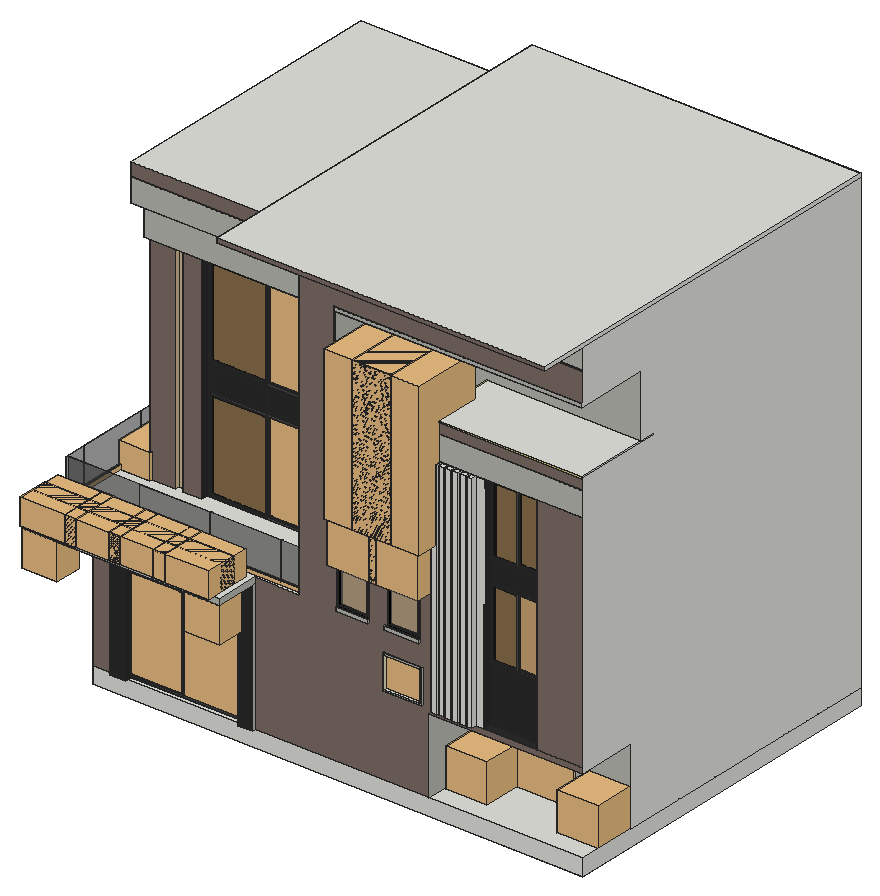
# SketchUp Ruby script. Lengths in inches.
U = 1.inch
M = Sketchup.active_model
def pt(a) = Geom::Point3d.new(a.map { |v| v * U })
def face(e, loops, mat)
  f = e.add_face(loops[0].map { |a| pt(a) })
  loops[1..].each { |l| e.add_face(l.map { |a| pt(a) }).erase! }
  f.material = f.back_material = mat if mat
  f
end
# faces: each face lists its corners as indices into pts; further lists are holes
def faces(e, pts, list, mat = nil) = list.each { |f| face(e, (f[0].is_a?(Array) ? f : [f]).map { |l| l.map { |i| pts[i] } }, mat) }
# xy, xz, yz: faces in a plane at the given z, y or x. An outline is a flat list of corners, or four numbers for a rectangle; further outlines are holes
def ring(l) = l.size == 4 ? [[l[0], l[1]], [l[2], l[1]], [l[2], l[3]], [l[0], l[3]]] : l.each_slice(2).to_a
def flat(e, list, mat, &to3) = list.each { |f| face(e, (f[0].is_a?(Array) ? f : [f]).map { |l| ring(l).map { |u, v| to3.(u, v) } }, mat) }
def xy(e, z, list, mat = nil) = flat(e, list, mat) { |x, y| [x, y, z] }
def xz(e, y, list, mat = nil) = flat(e, list, mat) { |x, z| [x, y, z] }
def yz(e, x, list, mat = nil) = flat(e, list, mat) { |y, z| [x, y, z] }
def lines(e, pts, list) = list.each { |a, b| e.add_line(pt(pts[a]), pt(pts[b])) }
# prism: a flat outline (further loops are holes) pulled along v
def prism(e, loops, v, mat = nil)
  f = face(e, loops, mat); d = Geom::Vector3d.new(v.map { |x| x * U })
  f.pushpull(f.normal.samedirection?(d) ? d.length : -d.length)
end
def box(e, o, s, mat = nil) = prism(e, [[o, [o[0] + s[0], o[1], o[2]], [o[0] + s[0], o[1] + s[1], o[2]], [o[0], o[1] + s[1], o[2]]]], [0, 0, s[2]], mat)
def at(x, y, z, deg = 0) = Geom::Transformation.translation(pt([x, y, z])) * Geom::Transformation.rotation(ORIGIN, Z_AXIS, deg.degrees)
def axes(o, x, y, z) = Geom::Transformation.new([*x, 0, *y, 0, *z, 0, *pt(o).to_a, 1])
def part(name) = M.definitions.add(name)
# library, detail: a bought-in or finely detailed component or shape, given as its bounding box
def library(name, o, s) = part(name).tap { |d| box(d.entities, o, s) }
def detail(e, o, s) = box(e.add_group.entities, o, s)
def put(e, d, t, mat = nil) = e.add_instance(d, t).tap { |i| i.material = mat if mat }
def group(e, t, mat = nil) = e.add_group.tap { |g| g.transformation = t; g.material = mat if mat }.entities
root = M.entities
M.materials.add("2").color = [128, 128, 128]
M.materials["2"].alpha = 0.5
M.materials.add("Glass_Tinted_Gray").color = [0, 0, 0]
M.materials["Glass_Tinted_Gray"].alpha = 0.125
M.materials.add("Lily_Light").color = [224, 224, 185]
M.materials.add("[0135_DarkGray]").color = [81, 81, 81]
M.materials.add("[0137_Black]").color = [0, 0, 0]
M.materials.add("[Color M07]").color = [43, 43, 43]
M.materials.add("[Color M08]").color = [30, 30, 30]
M.materials.add("[Formica Beige]").color = [211, 187, 149]
M.materials.add("[Mirror 02]").color = [229, 229, 229]
M.materials.add("[Terrazzo Light Blue]").color = [196, 214, 227]
M.materials.add("[Translucent_Glass_Blue]").color = [63, 63, 63]
M.materials["[Translucent_Glass_Blue]"].alpha = 0.35
M.materials.add("italian olive").color = [210, 204, 128]
M.materials.add("metal railing").color = [165, 165, 165]
M.materials.add("nimbu").color = [184, 186, 177]
M.materials.add("plastic2").color = [86, 86, 86]
M.materials.add("toasted toffee").color = [127, 111, 103]
c1 = part("PENTEK_RP Fineline 50S_Sliding_DoorCase_E1")
box(c1.entities,[0,0,0],[1.51,3.66,99.27],"[0135_DarkGray]")
c2 = part("PENTEK_RP Fineline 50S_SlidingDooe_Case_E2")
box(c2.entities,[0,0,0],[96.25,3.66,1.51],"[0135_DarkGray]")
c3 = part("pentek_RP Fineline 50S_SlidingDoor_Case")
put(c3.entities,c1,at(97.76,0,0))
put(c3.entities,c2,at(1.51,0,0))
put(c3.entities,c1,at(0,0,0))
put(c3.entities,c2,at(1.51,0,97.76))
c4 = part("PENTEK_RP Fineline 50S_SlidingDoor_GlazingBead_2")
box(c4.entities,[0,0,0],[0.56,0.59,94.39],"[0135_DarkGray]")
c5 = part("PENTEK_RP Fineline 50S_SlidingDoor_Glass")
box(c5.entities,[0,0,0],[46.58,0.16,94.39],"Glass_Tinted_Gray")
c6 = part("PENTEK_RP Fineline 50S_SlidingDoor_GlazingBead")
box(c6.entities,[0,0,0],[45.47,0.59,0.56],"[0135_DarkGray]")
c7 = part("PENTEK_RP Fineline 50S_SlidingDoor_Leaf_E1")
xy(c7.entities,0,[[0,0,0.93,1.97],[0.93,1.57,1.49,1.97]],"[0135_DarkGray]")
xy(c7.entities,96.25,[[0,0,0.93,0,0.93,1.57,1.49,1.57,1.49,1.97,0,1.97]],"[0135_DarkGray]")
xz(c7.entities,0,[[0,0,0.93,96.25]],"[0135_DarkGray]")
xz(c7.entities,1.57,[[0.93,0,1.49,95.32],[0.93,95.32,1.49,96.25]],"[0135_DarkGray]")
xz(c7.entities,1.97,[[0,0,1.49,96.25]],"[0135_DarkGray]")
yz(c7.entities,0,[[0,0,1.97,96.25]],"[0135_DarkGray]")
yz(c7.entities,0.93,[[0,0,1.57,0.93],[0,0.93,1.57,95.32],[0,95.32,1.57,96.25]],"[0135_DarkGray]")
yz(c7.entities,1.49,[[1.57,0,1.97,95.32],[1.57,95.32,1.97,96.25]],"[0135_DarkGray]")
c8 = part("PENTEK_RP Fineline 50S_SlidingDoor_Leaf_E2")
xy(c8.entities,0,[[0,0,0,1.57,0.56,1.57,0.56,1.97,46.02,1.97,46.02,1.57,46.58,1.57,46.58,0]],"[0135_DarkGray]")
xy(c8.entities,0.93,[[0,0,46.58,1.57]],"[0135_DarkGray]")
xy(c8.entities,1.49,[[0.56,1.57,46.02,1.97]],"[0135_DarkGray]")
xz(c8.entities,0,[[0,0,46.58,0.93]],"[0135_DarkGray]")
xz(c8.entities,1.57,[[0,0,0.56,0.93],[46.02,0,46.58,0.93],[0.56,0.93,46.02,1.49]],"[0135_DarkGray]")
xz(c8.entities,1.97,[[0.56,0,46.02,1.49]],"[0135_DarkGray]")
yz(c8.entities,0,[[0,0,1.57,0.93]],"[0135_DarkGray]")
yz(c8.entities,0.56,[[1.57,0,1.97,0.93],[1.57,0.93,1.97,1.49]],"[0135_DarkGray]")
yz(c8.entities,46.02,[[1.57,0,1.97,0.93],[1.57,0.93,1.97,1.49]],"[0135_DarkGray]")
yz(c8.entities,46.58,[[0,0,1.57,0.93]],"[0135_DarkGray]")
c9 = part("PENTEK_RP Fineline S_SlidingDoor_Leaf1")
put(c9.entities,c4,at(0.93,0,0.93))
put(c9.entities,c4,at(46.96,0,0.93))
put(c9.entities,c5,at(1.49,1.42,0.93))
put(c9.entities,c6,at(1.49,0,0.93))
put(c9.entities,c5,at(1.49,0.59,0.93),"[Terrazzo Light Blue]")
put(c9.entities,c7,at(0,0,0))
put(c9.entities,c7,axes([48.44,0,0],[-1,0,0],[0,1,0],[0,0,1]))
put(c9.entities,c8,axes([0.93,0,96.25],[1,0,0],[0,1,0],[0,0,-1]))
put(c9.entities,c8,at(0.93,0,0))
put(c9.entities,c6,at(1.49,0,94.77))
c10 = part("PENTEK_RP Fineline 50S_SlidingDoor_Leaf2")
put(c10.entities,c5,at(1.49,1.42,0.93))
put(c10.entities,c6,at(1.49,0,94.77))
put(c10.entities,c4,at(46.96,0,0.93))
put(c10.entities,c5,at(1.49,0.59,0.93),"[Mirror 02]")
put(c10.entities,c4,at(0.93,0,0.93))
put(c10.entities,c7,at(0,0,0))
put(c10.entities,c7,axes([48.44,0,0],[-1,0,0],[0,1,0],[0,0,1]))
put(c10.entities,c6,at(1.49,0,0.93))
put(c10.entities,c8,axes([0.93,0,96.25],[1,0,0],[0,1,0],[0,0,-1]))
put(c10.entities,c8,at(0.93,0,0))
c11 = part("PENTEK - Slimmest Steel Sliding Door / Window\#1")
put(c11.entities,c3,at(0,-1.88,-0.09))
put(c11.entities,c9,at(1.51,-2.27,1.42))
put(c11.entities,c10,at(49.32,-0.3,1.42))
c12 = part("Window black single")
xy(c12.entities,0,[[0,0,49.21,2.52]],"[0137_Black]")
xy(c12.entities,2.71,[[2.56,0,46.5,2.52]],"[0137_Black]")
xy(c12.entities,122.09,[[2.56,0,3.15,2.52],[3.15,0,46.5,2.52]],"[0137_Black]")
xy(c12.entities,124.8,[[0,0,49.21,2.52]],"[0137_Black]")
xz(c12.entities,0,[[[0,0,49.21,124.8],[2.56,2.71,46.5,122.09]]],"[0137_Black]")
xz(c12.entities,2.52,[[2.56,2.71,46.5,122.09]],"2")
xz(c12.entities,2.52,[[[0,0,49.21,124.8],[2.56,2.71,46.5,122.09]]],"[0137_Black]")
yz(c12.entities,0,[[0,0,2.52,2.71],[0,2.71,2.52,122.09],[0,122.09,2.52,124.8]],"[0137_Black]")
yz(c12.entities,2.56,[[0,2.71,2.52,122.09]],"[0137_Black]")
yz(c12.entities,46.5,[[0,2.71,2.52,122.09]],"[0137_Black]")
yz(c12.entities,49.21,[[0,0,2.52,124.8]],"[0137_Black]")
c13 = library("Railing",[0,0,0],[72,2.52,4.03])
c14 = part("railing plastic")
box(c14.entities,[0,0.75,0],[72,0.26,0.68],"plastic2")
box(c14.entities,[0,0,0],[72,0.26,0.68],"plastic2")
c15 = part("Glass Railing pro\#1")
put(c15.entities,c13,axes([0,0,0],[3.29426,0,0],[0,1,0],[0,0,1]))
put(c15.entities,c14,axes([0,0.75,3.47],[3.29426,0,0],[0,1,0],[0,0,1]))
c16 = part("sheet glass")
box(c16.entities,[0,0,0],[39.37,0.39,39.37],"[Translucent_Glass_Blue]")
c17 = part("glass stretch")
box(c17.entities,[0,0,0],[39.37,0.39,43.31],"[Translucent_Glass_Blue]")
c18 = part("glass frame\#1")
put(c18.entities,c16,axes([0,0,0],[1.8288,0,0],[0,1.016,0],[0,0,1]))
put(c18.entities,c17,axes([216.6,0,0],[0.52291,0,0],[0,1.016,0],[0,0,0.90909]))
put(c18.entities,c16,axes([72.2,0,0],[1.8288,0,0],[0,1.016,0],[0,0,1]))
put(c18.entities,c16,axes([144.4,0,0],[1.8288,0,0],[0,1.016,0],[0,0,1]))
c19 = part("Glass Railing +\#1")
put(c19.entities,c15,at(0,0,0),"metal railing")
put(c19.entities,c18,at(0,1.0625,1.53),"metal railing")
c20 = part("My+Glass_Railing\#1")
put(c20.entities,c19,at(-0.15,0,0))
c21 = part("Glass Railing pro")
put(c21.entities,c13,axes([0,0,0],[3.32754,0,0],[0,1,0],[0,0,1]))
put(c21.entities,c14,axes([0,0.75,3.47],[3.32754,0,0],[0,1,0],[0,0,1]))
c22 = part("glass frame")
put(c22.entities,c16,axes([0,0,0],[1.8288,0,0],[0,1.016,0],[0,0,1]))
put(c22.entities,c17,axes([216.6,0,0],[0.58376,0,0],[0,1.016,0],[0,0,0.90909]))
put(c22.entities,c16,axes([72.2,0,0],[1.8288,0,0],[0,1.016,0],[0,0,1]))
put(c22.entities,c16,axes([144.4,0,0],[1.8288,0,0],[0,1.016,0],[0,0,1]))
c23 = part("Glass Railing +")
put(c23.entities,c21,at(0,0,0),"metal railing")
put(c23.entities,c22,at(0,1.0625,1.53),"metal railing")
c24 = part("My+Glass_Railing")
put(c24.entities,c23,at(-0.16,0,0))
c25 = library("Pleated curtains",[0,0,0],[14.46,147.43,135.83])
c26 = library("My+Glass_Railing\#2",[-0.0625,0,0],[93.64,2.52,40.9])
c27 = library("Window with transom",[0,0,0],[5.2,55.12,70.87])
c28 = library("White+Curtain+Sketchup",[0,-2.58,0],[59,4.99,76.02])
c29 = library("Plante \#58",[-0.43,-1.58,0],[20.84,18.06,17.59])
c30 = library("Plant",[-27.84,-31.84,-1.26],[68.28,70.82,154.38])
c31 = library("climbing plant",[-30.01,-23.48,-50.28],[50.12,38.07,52.29])
c32 = library("Entrance door",[0,0,0],[60,4,84])
c33 = library("plant (1)",[-21.34,-27.21,-0.38],[41.91,41.15,38.97])
c34 = library("Group\#13",[0,0,0],[56.8,25.91,35.15])
xy(root,0,[[51.6,44.87,51.6,47.68,31.97,47.68,31.97,401.28,530.34,401.28,530.34,108.84,374.2,108.84,374.2,47.68,197.39,47.68,197.39,44.87,182.26,44.87,182.26,54.65,216.69,54.65,216.69,379.52,54.23,379.52,54.23,54.65,67.98,54.65,67.98,44.87]])
xy(root,76.96,[[374.2,47.68,530.34,108.84]])
xy(root,82.4,[[380.47,42.8,380.47,47.68,407.76,47.68,407.76,42.8,401.64,42.8,401.64,47.67,400.53,47.67,400.53,42.8,394.4,42.8,394.4,47.67,393.22,47.67,393.22,42.8,387.84,42.8,387.84,47.67,386.59,47.67,386.59,42.8],[409.39,42.8,415.51,47.68],[416.89,42.8,421.64,47.68]])
xy(root,82.4,[[430.39,47.68,483.63,56.54]],"[Color M07]")
xy(root,82.4,[[328.07,46.17,367.78,47.68]],"nimbu")
xy(root,83.48,[[431.47,56.54,455.45,56.85],[457.01,56.54,482.55,56.85]],"[Color M07]")
xy(root,83.98,[[329.65,46.17,366.19,74.5]])
xy(root,100.15,[[67.98,48.03,67.98,54.65,54.23,54.65,54.23,379.52,216.69,379.52,216.69,54.65,182.26,54.65,182.26,48.03]])
xy(root,115.19,[[329.65,46.17,366.19,74.5]],"Lily_Light")
xy(root,116.77,[[328.07,46.17,367.78,47.68]])
xy(root,133.04,[[0,2.67,0,401.28,31.97,401.28,31.97,47.68,51.6,47.68,51.6,44.87,67.98,44.87,67.98,48.03,182.26,48.03,182.26,44.87,197.39,44.87,197.39,2.67]],"nimbu")
xy(root,138.04,[[280.61,46.18,313.3,47.68],[280.61,47.68,313.3,163.48],[329.73,47.68,364.78,163.48]])
xy(root,138.04,[[329.73,46.18,364.78,47.68]],"nimbu")
xy(root,138.65,[[431.47,56.54,455.45,56.85],[457.01,56.54,482.55,56.85]],"[Color M07]")
xy(root,139.14,[[0,2.67,197.39,2.67,197.39,47.68,242.11,47.68,242.11,117.14,206.54,117.14,85.61,120.06,65.875,120.06,65.875,124.29,58.79,124.29,58.79,120.06,31.97,120.06,31.97,172.94,85.61,172.94,85.61,120.06,206.54,117.14,206.54,296.25,28.11,296.25,28.11,304.8,48.45,304.8,48.45,357.56,28.11,357.56,28.11,401.28,0,401.28]])
xy(root,139.73,[[430.39,56.54,483.63,56.54,483.63,56.85,500.01,56.85,500.01,164.99,280.61,164.99,280.61,56.79,329.73,56.79,364.78,56.85,430.39,56.85]])
xy(root,141.67,[[280.61,46.18,313.3,56.79]])
xy(root,141.79,[[329.73,46.18,364.78,46.18,364.78,56.85,329.73,56.79,332.17,56.79,332.17,47.68,329.73,47.68]])
xy(root,211.71,[[280.61,47.68,280.61,164.99,500.01,164.99,500.01,56.85,483.63,56.85,483.63,56.54,430.39,56.54,430.39,56.85,364.78,56.85,364.78,47.68,332.17,47.68,332.17,56.79,313.3,56.79,313.3,47.68]])
xy(root,212.79,[[431.47,56.54,455.45,56.85],[457.01,56.54,482.55,56.85]],"[Color M07]")
xy(root,233.46,[[431.47,56.54,455.45,56.85],[457.01,56.54,482.55,56.85]],"[Color M07]")
xy(root,234.49,[[277.8,46.875,374.2,47.68]])
xy(root,234.54,[[430.39,56.54,483.63,56.54,483.63,56.85,500.01,56.85,500.01,164.99,410.45,164.99,410.45,56.85,430.39,56.85]])
xy(root,234.56,[[85.61,127.3,85.61,172.94,35.22,172.94,35.22,296.25,206.54,296.25,206.54,127.3]])
xy(root,237.16,[[280.61,46.875,374.2,122.34]])
xy(root,237.7,[[88.75,126.36,146.08,127.3],[148.58,126.36,203.4,127.3]])
xy(root,257.93,[[88.75,126.36,146.08,127.3],[148.58,126.36,203.4,127.3]])
xy(root,261.07,[[85.61,127.3,206.54,127.3,206.54,155.49,241.84,155.49,241.84,296.25,35.22,296.25,35.22,172.94,85.61,172.94]])
xy(root,309.83,[[380.47,42.8,386.59,42.8,386.59,47.67,387.84,47.67,387.84,42.8,393.22,42.8,393.22,47.67,394.4,47.67,394.4,42.8,400.53,42.8,400.53,47.67,401.64,47.67,401.64,42.8,407.76,42.8,407.76,47.68,409.39,47.68,409.39,42.8,415.51,42.8,415.51,47.68,416.89,47.68,416.89,42.8,421.64,42.8,421.64,47.87,380.97,47.87,380.97,47.68,380.47,47.68],[483.63,47.68,530.34,47.87]])
xy(root,309.83,[[430.39,47.87,430.39,56.85,410.45,56.85,410.45,164.99,500.01,164.99,500.01,56.85,483.63,56.85,483.63,47.87]],"[Color M07]")
xy(root,309.83,[[374.2,47.68,380.97,47.68,380.97,47.87,374.39,47.87,374.39,122.34,374.2,122.34]],"toasted toffee")
xy(root,310.55,[[374.2,47.68,374.2,122.34,374.39,122.34,374.39,47.87,530.34,47.87,530.34,47.68]])
xy(root,335.16,[[374.2,47.68,374.39,122.34],[374.39,47.68,530.34,47.87]])
xy(root,335.9,[[374.2,47.68,374.2,122.34,374.39,122.34,374.39,47.87,530.34,47.87,530.34,47.68]],"toasted toffee")
xy(root,346.22,[[373.53,46.625,373.53,122.34,374.2,122.34,374.2,47.68,530.34,47.68,530.34,46.625],[374.2,47.68,530.34,138.03],[373.53,122.34,374.2,138.03]])
xy(root,347.63,[[373.53,46.625,530.34,122.34],[373.53,122.34,530.34,138.03]])
xy(root,359.34,[[206.54,155.49,206.54,172.94,35.22,172.94,35.22,296.25,241.84,296.25,241.84,155.49]])
xy(root,359.34,[[28.11,117.14,28.11,172.94,31.97,172.94,31.97,120.06,58.79,120.06,58.79,124.29,65.875,124.29,65.875,120.06,85.61,120.06,85.61,172.94,206.54,172.94,206.54,117.14],[28.11,172.94,35.22,296.25],[28.11,304.8,48.45,357.56]],"nimbu")
xy(root,392.4,[[22.03,108.47,22.03,401.28,28.11,401.28,28.11,117.14,242.11,117.14,242.11,108.47]],"nimbu")
xy(root,410.95,[[280.61,46.875,530.34,122.34]])
xy(root,414.45,[[277.8,46.875,530.34,47.68]],"italian olive")
xy(root,415.9,[[22.03,108.47,242.11,108.47,242.11,110.27,23.83,110.27,23.83,401.28,22.03,401.28]])
xy(root,416.63,[[22.03,108.47,22.03,401.28,23.83,401.28,23.83,110.27,242.11,110.27,242.11,108.47]],"toasted toffee")
xy(root,429.77,[[22.03,108.47,242.11,401.28]])
xy(root,443.41,[[242.11,47.68,530.34,47.68,530.34,48.63,243.0625,48.63,243.0625,401.28,242.11,401.28]])
xy(root,445.02,[[242.11,47.68,242.11,401.28,243.0625,401.28,243.0625,48.63,530.34,48.63,530.34,47.68]],"nimbu")
xy(root,464.8,[[196.3,0,196.3,401.28,242.11,401.28,242.11,47.68,530.34,47.68,530.34,0],[242.11,47.68,530.34,401.28]])
xy(root,469.04,[[196.3,0,530.34,401.28]])
xz(root,0,[[196.3,464.8,530.34,469.04]],"toasted toffee")
xz(root,2.67,[[0,133.04,197.39,139.14]],"nimbu")
xz(root,42.8,[[380.47,82.4,386.59,309.83],[387.84,82.4,393.22,309.83],[394.4,82.4,400.53,309.83],[401.64,82.4,407.76,309.83],[409.39,82.4,415.51,309.83],
  [416.89,82.4,421.64,309.83]])
xz(root,44.87,[[51.6,0,67.98,133.04],[182.26,0,197.39,133.04]],"[Color M07]")
xz(root,46.17,[[[328.07,82.4,367.78,116.77],[329.65,83.98,366.19,115.19]]],"nimbu")
xz(root,46.18,[[280.61,138.04,313.3,141.67],[329.73,138.04,364.78,141.79]],"nimbu")
xz(root,46.625,[[373.53,346.22,530.34,347.63]],"italian olive")
xz(root,46.875,[[277.8,234.49,374.2,234.49,374.2,237.16,280.61,237.16,280.61,410.95,530.34,410.95,530.34,414.45,277.8,414.45]],"nimbu")
xz(root,47.67,[[386.59,82.4,387.84,309.83],[393.22,82.4,394.4,309.83],[400.53,82.4,401.64,309.83]])
xz(root,47.68,[[407.76,82.4,409.39,309.83],[415.51,82.4,416.89,309.83]])
xz(root,47.68,[[374.2,310.55,530.34,335.16],[242.11,445.02,530.34,464.8]],"nimbu")
xz(root,47.68,[[31.97,0,51.6,133.04],[[197.39,0,374.2,0,374.2,76.96,530.34,76.96,530.34,82.4,328.07,82.4,328.07,116.77,367.78,116.77,367.78,82.4,380.47,82.4,380.47,211.71,364.78,211.71,364.78,138.04,329.73,138.04,329.73,141.79,332.17,141.79,332.17,211.71,380.47,211.71,380.47,309.83,374.2,309.83,374.2,234.49,277.8,234.49,277.8,414.45,530.34,414.45,530.34,443.41,242.11,443.41,242.11,139.14,197.39,139.14],[280.61,138.04,313.3,211.71]],[483.63,82.4,530.34,309.83],[374.2,335.9,530.34,346.22]],"toasted toffee")
xz(root,47.87,[[374.39,309.83,530.34,310.55],[374.39,335.16,530.34,335.9]])
xz(root,48.03,[[67.98,100.15,182.26,133.04]],"[Color M07]")
xz(root,48.63,[[243.0625,443.41,530.34,445.02]],"nimbu")
xz(root,54.65,[[54.23,0,67.98,100.15],[182.26,0,216.69,100.15]])
xz(root,56.54,[[[430.39,82.4,483.63,139.73],[431.47,83.48,482.55,138.65]],[455.45,83.48,457.01,138.65],[[430.39,211.71,483.63,234.54],[431.47,212.79,482.55,233.46]],[455.45,212.79,457.01,233.46]],"[Color M07]")
xz(root,56.79,[[280.61,139.73,313.3,141.67],[313.3,139.73,313.3,211.71,332.17,211.71,332.17,141.79,329.73,141.79,329.73,139.73]])
xz(root,56.85,[[364.78,139.73,430.39,211.71],[483.63,139.73,500.01,211.71],[410.45,234.54,430.39,309.83],[483.63,234.54,500.01,309.83]])
xz(root,56.85,[[431.47,83.48,455.45,138.65],[457.01,83.48,482.55,138.65],[431.47,212.79,455.45,233.46],[457.01,212.79,482.55,233.46]],"[Color M07]")
xz(root,74.5,[[329.65,83.98,366.19,115.19]],"Lily_Light")
xz(root,108.47,[[22.03,392.4,242.11,415.9]],"nimbu")
xz(root,108.47,[[22.03,416.63,242.11,429.77]],"toasted toffee")
xz(root,108.84,[[374.2,0,530.34,76.96]],"nimbu")
xz(root,110.27,[[23.83,415.9,242.11,416.63]])
xz(root,117.14,[[28.11,359.34,242.11,392.4]],"nimbu")
xz(root,117.14,[[206.54,139.14,242.11,359.34]],"toasted toffee")
xz(root,120.06,[[31.97,139.14,58.79,359.34],[65.875,139.14,85.61,359.34]],"toasted toffee")
xz(root,122.34,[[280.61,237.16,374.2,237.16,374.2,309.83,374.39,309.83,374.39,310.55,374.2,310.55,374.2,335.16,374.39,335.16,374.39,335.9,374.2,335.9,374.2,346.22,373.53,346.22,373.53,347.63,530.34,347.63,530.34,410.95,280.61,410.95]],"nimbu")
xz(root,124.29,[[58.79,139.14,65.875,359.34]],"[Formica Beige]")
xz(root,126.36,[[88.75,237.7,146.08,257.93],[148.58,237.7,203.4,257.93]],"[Color M07]")
xz(root,127.3,[[[85.61,234.56,206.54,261.07],[88.75,237.7,203.4,257.93]],[146.08,237.7,148.58,257.93]],"[Color M07]")
xz(root,138.03,[[373.53,346.22,530.34,347.63]])
xz(root,155.49,[[206.54,261.07,241.84,359.34]])
xz(root,164.99,[[410.45,234.54,500.01,309.83]])
xz(root,164.99,[[280.61,139.73,500.01,211.71]],"Lily_Light")
xz(root,172.94,[[31.97,139.14,31.97,359.34,85.61,359.34,85.61,261.07,35.22,261.07,35.22,234.56,85.61,234.56,85.61,139.14]],"[Color M08]")
xz(root,296.25,[[35.22,234.56,35.58,234.56,35.51,261.07,35.22,261.07]])
xz(root,296.25,[[35.86,139.14,206.54,139.14,206.54,234.56,35.58,234.56],[35.51,261.07,241.84,261.07,241.84,359.34,35.22,359.34]],"Lily_Light")
xz(root,296.25,[[28.11,139.14,35.86,139.14,35.58,234.56,35.22,234.56,35.22,261.07,35.51,261.07,35.22,359.34,28.11,359.34]],"[Color M08]")
xz(root,304.8,[[28.11,139.14,48.45,359.34]],"nimbu")
xz(root,357.56,[[28.11,139.14,48.45,359.34]],"toasted toffee")
xz(root,379.52,[[54.23,0,216.69,100.15]],"Lily_Light")
xz(root,401.28,[[31.97,0,31.97,133.04,0,133.04,0,139.14,28.11,139.14,28.11,392.4,22.03,392.4,22.03,415.9,23.83,415.9,23.83,416.63,22.03,416.63,22.03,429.77,242.11,429.77,242.11,419.81,530.34,419.81,530.34,0],[242.11,419.81,242.11,443.41,243.0625,443.41,243.0625,445.02,242.11,445.02,242.11,464.8,530.34,464.8,530.34,419.81],[196.3,464.8,530.34,469.04]])
yz(root,0,[[2.67,133.04,401.28,139.14]],"nimbu")
yz(root,22.03,[[108.47,392.4,401.28,415.9]],"nimbu")
yz(root,22.03,[[108.47,416.63,401.28,429.77]],"toasted toffee")
yz(root,23.83,[[110.27,415.9,401.28,416.63]])
yz(root,28.11,[[117.14,359.34,401.28,392.4]],"nimbu")
yz(root,28.11,[[296.25,139.14,304.8,359.34],[357.56,139.14,401.28,359.34]],"toasted toffee")
yz(root,31.97,[[47.68,0,401.28,133.04],[120.06,139.14,172.94,359.34]],"toasted toffee")
yz(root,35.22,[[172.94,234.56,296.25,261.07]],"[Color M07]")
yz(root,48.45,[[304.8,139.14,357.56,359.34]],"nimbu")
yz(root,51.6,[[44.87,0,47.68,133.04]],"[Color M07]")
yz(root,54.23,[[54.65,0,379.52,100.15]],"Lily_Light")
yz(root,58.79,[[120.06,139.14,124.29,359.34]],"[Formica Beige]")
yz(root,65.875,[[120.06,139.14,124.29,359.34]],"[Formica Beige]")
yz(root,67.98,[[44.87,0,54.65,0,54.65,100.15,48.03,100.15,48.03,133.04,44.87,133.04]],"[Color M07]")
yz(root,85.61,[[127.3,139.14,172.94,234.56],[127.3,261.07,172.94,359.34]])
yz(root,85.61,[[120.06,139.14,127.3,359.34]],"[Color M07]")
yz(root,88.75,[[126.36,237.7,127.3,257.93]])
yz(root,146.08,[[126.36,237.7,127.3,257.93]],"[Color M07]")
yz(root,148.58,[[126.36,237.7,127.3,257.93]],"[Color M07]")
yz(root,182.26,[[44.87,0,44.87,133.04,48.03,133.04,48.03,100.15,54.65,100.15,54.65,0]],"[Color M07]")
yz(root,196.3,[[0,464.8,401.28,469.04]],"toasted toffee")
yz(root,197.39,[[44.87,0,47.68,133.04],[2.67,133.04,47.68,139.14]],"nimbu")
yz(root,203.4,[[126.36,237.7,127.3,257.93]])
yz(root,206.54,[[127.3,139.14,296.25,234.56],[127.3,261.07,155.49,359.34]],"Lily_Light")
yz(root,206.54,[[117.14,139.14,127.3,359.34]],"[Color M07]")
yz(root,216.69,[[54.65,0,379.52,100.15]],"Lily_Light")
yz(root,241.84,[[155.49,261.07,296.25,359.34]],"Lily_Light")
yz(root,242.11,[[47.68,445.02,401.28,464.8]],"nimbu")
yz(root,242.11,[[47.68,139.14,47.68,443.41,401.28,443.41,401.28,429.77,108.47,429.77,108.47,416.63,110.27,416.63,110.27,415.9,108.47,415.9,108.47,392.4,117.14,392.4,117.14,139.14]],"toasted toffee")
yz(root,243.0625,[[48.63,443.41,401.28,445.02]],"nimbu")
yz(root,277.8,[[46.875,234.49,47.68,414.45]],"italian olive")
yz(root,280.61,[[47.68,138.04,163.48,138.04,163.48,139.73,56.79,139.73,56.79,141.67,47.68,141.67]])
yz(root,280.61,[[56.79,139.73,164.99,139.73,164.99,211.71,47.68,211.71,47.68,141.67,56.79,141.67]],"Lily_Light")
yz(root,280.61,[[46.18,138.04,47.68,141.67],[46.875,237.16,122.34,410.95]],"nimbu")
yz(root,313.3,[[47.68,141.67,56.79,211.71]])
yz(root,313.3,[[46.18,138.04,47.68,141.67]],"nimbu")
yz(root,328.07,[[46.17,82.4,47.68,116.77]],"nimbu")
yz(root,329.65,[[46.17,83.98,74.5,115.19]],"Lily_Light")
yz(root,329.73,[[46.18,138.04,47.68,141.79]],"nimbu")
yz(root,332.17,[[47.68,141.79,56.79,211.71]])
yz(root,364.78,[[47.68,141.79,56.85,211.71]])
yz(root,364.78,[[46.18,138.04,47.68,141.79]],"nimbu")
yz(root,366.19,[[46.17,83.98,74.5,115.19]],"Lily_Light")
yz(root,367.78,[[46.17,82.4,47.68,116.77]],"nimbu")
yz(root,373.53,[[122.34,346.22,138.03,347.63]])
yz(root,373.53,[[46.625,346.22,122.34,347.63]],"italian olive")
yz(root,374.2,[[46.875,234.49,47.68,237.16]])
yz(root,374.2,[[47.68,0,108.84,76.96],[47.68,310.55,122.34,335.16]],"nimbu")
yz(root,374.2,[[47.68,237.16,122.34,309.83],[47.68,335.9,122.34,346.22]],"toasted toffee")
yz(root,374.39,[[47.87,309.83,122.34,310.55],[47.87,335.16,122.34,335.9]])
yz(root,380.47,[[42.8,82.4,47.68,309.83]])
yz(root,386.59,[[42.8,82.4,47.67,309.83]])
yz(root,387.84,[[42.8,82.4,47.67,309.83]])
yz(root,393.22,[[42.8,82.4,47.67,309.83]])
yz(root,394.4,[[42.8,82.4,47.67,309.83]])
yz(root,400.53,[[42.8,82.4,47.67,309.83]])
yz(root,401.64,[[42.8,82.4,47.67,309.83]])
yz(root,407.76,[[42.8,82.4,47.68,309.83]])
yz(root,409.39,[[42.8,82.4,47.68,309.83]])
yz(root,410.45,[[56.85,234.54,164.99,309.83]])
yz(root,415.51,[[42.8,82.4,47.68,309.83]])
yz(root,416.89,[[42.8,82.4,47.68,309.83]])
yz(root,421.64,[[42.8,82.4,47.68,82.4,47.87,309.83,42.8,309.83]])
yz(root,430.39,[[47.68,82.4,56.54,82.4,56.54,139.73,56.85,139.73,56.85,211.71,56.54,211.71,56.54,234.54,56.85,234.54,56.85,309.83,47.87,309.83]],"[Color M07]")
yz(root,431.47,[[56.54,83.48,56.85,138.65],[56.54,212.79,56.85,233.46]],"[Color M07]")
yz(root,455.45,[[56.54,83.48,56.85,138.65],[56.54,212.79,56.85,233.46]],"[Color M07]")
yz(root,457.01,[[56.54,83.48,56.85,138.65],[56.54,212.79,56.85,233.46]],"[Color M07]")
yz(root,482.55,[[56.54,83.48,56.85,138.65],[56.54,212.79,56.85,233.46]],"[Color M07]")
yz(root,483.63,[[47.68,82.4,47.68,309.83,56.85,309.83,56.85,234.54,56.54,234.54,56.54,211.71,56.85,211.71,56.85,139.73,56.54,139.73,56.54,82.4]],"[Color M07]")
yz(root,500.01,[[56.85,234.54,164.99,309.83]])
yz(root,500.01,[[56.85,139.73,164.99,211.71]],"Lily_Light")
yz(root,530.34,[[108.84,0,401.28,0,401.28,464.8,47.68,464.8,47.68,445.02,48.63,445.02,48.63,443.41,47.68,443.41,47.68,414.45,46.875,414.45,46.875,410.95,122.34,410.95,122.34,347.63,138.03,347.63,138.03,346.22,47.68,346.22,47.68,335.9,47.87,335.9,47.87,335.16,47.68,335.16,47.68,310.55,47.87,310.55,47.87,309.83,47.68,309.83,47.68,76.96,108.84,76.96],[46.625,346.22,138.03,347.63],[0,464.8,401.28,469.04]])
p = [[421.64,47.87,309.83],[421.64,47.68,82.4],[430.39,47.68,82.4],[430.39,47.87,309.83],[364.78,56.85,139.73],[329.73,56.79,139.73],
  [329.73,56.79,141.79],[364.78,56.85,141.79]]
faces(root,p,[[0,1,2,3],[4,5,6,7]])
put(root,c11,axes([85.61,129.17,261.16],[1.2182,0,0],[0,1,0],[0,0,0.99]))
put(root,c11,axes([85.61,129.17,139.23],[1.2182,0,0],[0,1,0],[0,0,0.9603]))
put(root,c11,axes([430.42,58.42,234.61],[0.53601,0,0],[0,1,0],[0,0,0.75848]))
put(root,c11,axes([430.42,58.42,139.8],[0.53601,0,0],[0,1,0],[0,0,0.72513]))
put(root,c11,axes([37.49,296.26,261.15],[0.00419,-1.24203,0],[0.99999,0.00338,0],[0,0,0.99]))
put(root,c11,axes([36.68,296.25,139.23],[0.00419,-1.24203,0],[0.99999,0.00338,0],[0,0,0.96115]))
put(root,c12,axes([28.11,357.56,139.14],[0,-1.07219,0],[1,0,0],[0,0,1.76439]))
put(root,c20,at(5.07,49.92,139.14))
put(root,c24,at(2.35,289.35,139.125,-90))
put(root,c25,axes([206.51,128.87,261.07],[0,0.56,0],[-0.82,0,0],[0,0,0.7235]))
put(root,c25,axes([206.51,128.87,136.2],[0,0.56,0],[-0.82,0,0],[0,0,0.7235]))
put(root,c25,axes([37.58,180.86,264.03],[0.56,0,0],[0,0.82,0],[0,0,0.7235]))
put(root,c25,axes([40.78,172.94,139.14],[0.56,0,0],[0,0.82,0],[0,0,0.7018]))
put(root,c26,at(280.62,47.68,237.15))
put(root,c12,axes([280.61,47.68,141.67],[0.6642,0,0],[0,1,0],[0,0,0.5612]))
put(root,c12,axes([332.09,47.68,141.79],[0.6642,0,0],[0,1,0],[0,0,0.5612]))
put(root,c27,axes([366.17,49.02,83.9375],[0,0.10269,0],[-0.66306,0,0],[0,0,0.42844]))
put(root,c28,axes([432.03,62.67,231.55],[0.84741,0,0],[0,1,0],[0,0,1.01486]))
put(root,c28,axes([432.03,61.29,134.21],[0.85751,0,0],[0,1,0],[0,0,1.01486]))
put(root,c28,axes([282.3125,53,139.73],[0.52521,0,0],[0,0.50507,0],[0,0,0.94687]))
put(root,c28,axes([332.43,53,139.73],[0.52521,0,0],[0,0.50507,0],[0,0,0.94687]))
put(root,c29,axes([-3.41,5.03,96.89],[1.73356,0,0],[0,1.5,0],[0,0,2.055]))
put(root,c29,axes([162.01,5.03,96.89],[1.73356,0,0],[0,1.5,0],[0,0,2.055]))
put(root,c30,at(343.88,54.43,236.47))
put(root,c30,at(314.88,54.43,236.47))
put(root,c31,at(355.94,55.3125,237.16))
put(root,c31,at(312.57,55.3125,237.16))
put(root,c32,axes([414.63,105.96,0],[1,0,0],[0,0.58,0],[0,0,0.79709]))
put(root,c33,at(396.35,95.32,0))
put(root,c33,at(509.77,95.32,0))
put(root,c11,axes([61.32,52.87,1.96],[1.2182,0,0],[0,1,0],[0,0,0.99]))
put(root,c25,axes([60.9,59.09,0.88],[0,-0.56,0],[0.82,0,0],[0,0,0.7235]))
put(root,c34,axes([-0.71,-3.52,139.14],[1,0,0],[0,1.22347,0],[0,0,0.73]))
put(root,c34,axes([-0.71,12.35,139.14],[1,0,0],[0,1.22347,0],[0,0,0.73]))
put(root,c34,axes([44.24,-3.52,139.14],[1,0,0],[0,1.22347,0],[0,0,0.73]))
put(root,c34,axes([44.24,12.35,139.14],[1,0,0],[0,1.22347,0],[0,0,0.73]))
put(root,c34,axes([89.4,-3.52,139.14],[1,0,0],[0,1.22347,0],[0,0,0.73]))
put(root,c34,axes([89.4,12.35,139.14],[1,0,0],[0,1.22347,0],[0,0,0.73]))
put(root,c34,axes([134.35,-3.52,139.14],[1,0,0],[0,1.22347,0],[0,0,0.73]))
put(root,c34,axes([134.35,12.35,139.14],[1,0,0],[0,1.22347,0],[0,0,0.73]))
put(root,c34,axes([34.05,117.55,139.14],[0,1,0],[-1.22347,0,0],[0,0,0.73]))
put(root,c34,axes([34.05,252.62,139.14],[0,1,0],[-1.22347,0,0],[0,0,0.73]))
put(root,c34,axes([34.05,207.66,139.14],[0,1,0],[-1.22347,0,0],[0,0,0.73]))
put(root,c34,axes([34.05,162.51,139.14],[0,1,0],[-1.22347,0,0],[0,0,0.73]))
g1 = group(root,at(31.97,401.28,-16.57))
box(g1,[0,-353.6,0],[498.37,353.6,16.57])
